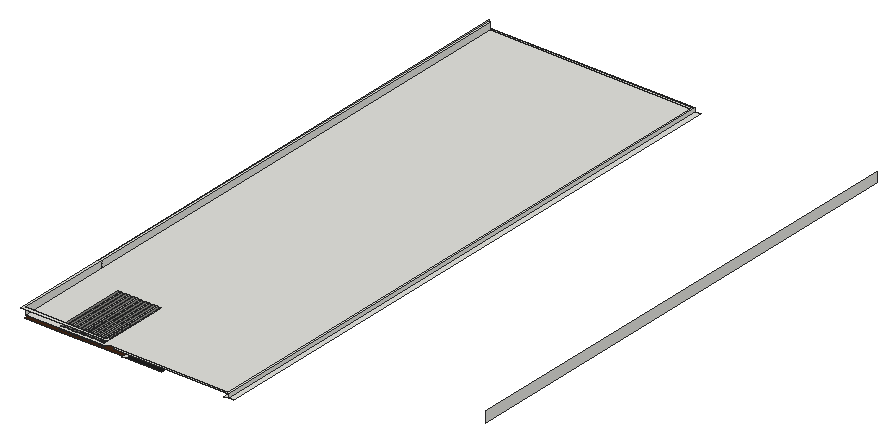
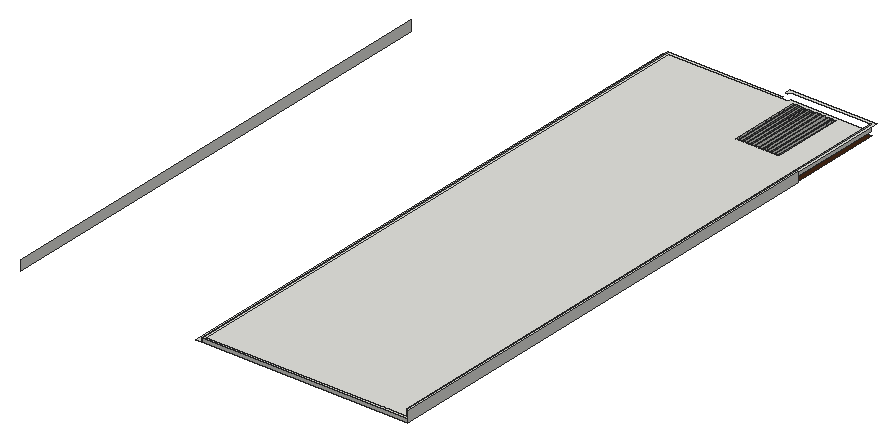
# SketchUp Ruby script. Lengths in inches.
U = 1.inch
M = Sketchup.active_model
def pt(a) = Geom::Point3d.new(a.map { |v| v * U })
def face(e, loops, mat)
  f = e.add_face(loops[0].map { |a| pt(a) })
  loops[1..].each { |l| e.add_face(l.map { |a| pt(a) }).erase! }
  f.material = f.back_material = mat if mat
  f
end
# faces: each face lists its corners as indices into pts; further lists are holes
def faces(e, pts, list, mat = nil) = list.each { |f| face(e, (f[0].is_a?(Array) ? f : [f]).map { |l| l.map { |i| pts[i] } }, mat) }
# xy, xz, yz: faces in a plane at the given z, y or x. An outline is a flat list of corners, or four numbers for a rectangle; further outlines are holes
def ring(l) = l.size == 4 ? [[l[0], l[1]], [l[2], l[1]], [l[2], l[3]], [l[0], l[3]]] : l.each_slice(2).to_a
def flat(e, list, mat, &to3) = list.each { |f| face(e, (f[0].is_a?(Array) ? f : [f]).map { |l| ring(l).map { |u, v| to3.(u, v) } }, mat) }
def xy(e, z, list, mat = nil) = flat(e, list, mat) { |x, y| [x, y, z] }
def xz(e, y, list, mat = nil) = flat(e, list, mat) { |x, z| [x, y, z] }
def yz(e, x, list, mat = nil) = flat(e, list, mat) { |y, z| [x, y, z] }
def lines(e, pts, list) = list.each { |a, b| e.add_line(pt(pts[a]), pt(pts[b])) }
# prism: a flat outline (further loops are holes) pulled along v
def prism(e, loops, v, mat = nil)
  f = face(e, loops, mat); d = Geom::Vector3d.new(v.map { |x| x * U })
  f.pushpull(f.normal.samedirection?(d) ? d.length : -d.length)
end
def box(e, o, s, mat = nil) = prism(e, [[o, [o[0] + s[0], o[1], o[2]], [o[0] + s[0], o[1] + s[1], o[2]], [o[0], o[1] + s[1], o[2]]]], [0, 0, s[2]], mat)
def at(x, y, z, deg = 0) = Geom::Transformation.translation(pt([x, y, z])) * Geom::Transformation.rotation(ORIGIN, Z_AXIS, deg.degrees)
def axes(o, x, y, z) = Geom::Transformation.new([*x, 0, *y, 0, *z, 0, *pt(o).to_a, 1])
def part(name) = M.definitions.add(name)
# library, detail: a bought-in or finely detailed component or shape, given as its bounding box
def library(name, o, s) = part(name).tap { |d| box(d.entities, o, s) }
def detail(e, o, s) = box(e.add_group.entities, o, s)
def put(e, d, t, mat = nil) = e.add_instance(d, t).tap { |i| i.material = mat if mat }
def group(e, t, mat = nil) = e.add_group.tap { |g| g.transformation = t; g.material = mat if mat }.entities
root = M.entities
M.materials.add("[Color M08]").color = [30, 30, 30]
M.materials.add("[Field Square Tile]").color = [211, 167, 108]
M.materials.add("[Granite Light Gray]").color = [149, 148, 144]
M.materials.add("[Wood Veneer 01]").color = [66, 38, 20]
xy(root,380.5,[[676.54,2346.71,676.54,3661.44,228.78,3661.44,228.78,2597.8,444.78,2597.8,444.78,2562.82,218.97,2562.82,218.97,3671.25,686.35,3671.25,686.35,2346.71],[444.78,2346.71,453.7,2425.46],[686.35,2346.71,698.16,3671.25],[444.78,2425.46,444.78,2597.8,228.78,2597.8,228.78,3661.44,676.54,3661.44,676.54,2425.46,629.77,2425.46,629.77,2532.83,534.46,2532.83,534.46,2573.65,453.7,2573.65,453.7,2532.83,445.08,2532.83,445.08,2425.46],[445.08,2425.46,453.7,2532.83],
  [534.46,2425.46,629.77,2532.83],[453.7,2532.83,534.46,2573.65]])
xy(root,380.5,[[453.7,2346.71,534.46,2532.83]],"[Color M08]")
xy(root,380.5,[[[223.8,2347.9,295.73,2562.82],[240.83,2441.63,242.35,2442.01,243.73,2442.76,244.86,2443.84,245.67,2445.18,246.1,2446.6875,246.14,2448.25,245.76,2449.78,245.01,2451.15,243.92,2452.28,242.58,2453.09,241.08,2453.53,239.51,2453.56,237.99,2453.19,236.62,2452.43,235.49,2451.35,234.68,2450.01,234.24,2448.5,234.21,2446.9375,234.58,2445.41,235.34,2444.04,236.42,2442.91,237.76,2442.1,239.27,2441.66],[240.83,2389.88,242.35,2390.26,243.73,2391.01,244.86,2392.09,245.67,2393.43,246.1,2394.9375,246.14,2396.5,245.76,2398.03,245.01,2399.4,243.92,2400.53,242.58,2401.34,241.08,2401.78,239.51,2401.81,237.99,2401.44,236.62,2400.68,235.49,2399.6,234.68,2398.26,234.24,2396.75,234.21,2395.1875,234.58,2393.66,235.34,2392.29,236.42,2391.16,237.76,2390.35,239.27,2389.91],[240.83,2359.13,242.35,2359.51,243.73,2360.26,244.86,2361.34,245.67,2362.68,246.1,2364.1875,246.14,2365.75,245.76,2367.28,245.01,2368.65,243.92,2369.78,242.58,2370.59,241.08,2371.03,239.51,2371.06,237.99,2370.69,236.62,2369.93,235.49,2368.85,234.68,2367.51,234.24,2366,234.21,2364.4375,234.58,2362.91,235.34,2361.54,236.42,2360.41,237.76,2359.6,239.27,2359.16],[240.83,2501.63,242.35,2502.01,243.73,2502.76,244.86,2503.84,245.67,2505.18,246.1,2506.6875,246.14,2508.25,245.76,2509.78,245.01,2511.15,243.92,2512.28,242.58,2513.09,241.08,2513.53,239.51,2513.56,237.99,2513.19,236.62,2512.43,235.49,2511.35,234.68,2510.01,234.24,2508.5,234.21,2506.9375,234.58,2505.41,235.34,2504.04,236.42,2502.91,237.76,2502.1,239.27,2501.66],[280.58,2501.63,282.1,2502.01,283.48,2502.76,284.61,2503.84,285.42,2505.18,285.85,2506.6875,285.89,2508.25,285.51,2509.78,284.76,2511.15,283.67,2512.28,282.33,2513.09,280.83,2513.53,279.26,2513.56,277.74,2513.19,276.37,2512.43,275.24,2511.35,274.43,2510.01,273.99,2508.5,273.96,2506.9375,274.33,2505.41,275.09,2504.04,276.17,2502.91,277.51,2502.1,279.02,2501.66],[280.58,2441.63,282.1,2442.01,283.48,2442.76,284.61,2443.84,285.42,2445.18,285.85,2446.6875,285.89,2448.25,285.51,2449.78,284.76,2451.15,283.67,2452.28,282.33,2453.09,280.83,2453.53,279.26,2453.56,277.74,2453.19,276.37,2452.43,275.24,2451.35,274.43,2450.01,273.99,2448.5,273.96,2446.9375,274.33,2445.41,275.09,2444.04,276.17,2442.91,277.51,2442.1,279.02,2441.66],[280.58,2389.88,282.1,2390.26,283.48,2391.01,284.61,2392.09,285.42,2393.43,285.85,2394.9375,285.89,2396.5,285.51,2398.03,284.76,2399.4,283.67,2400.53,282.33,2401.34,280.83,2401.78,279.26,2401.81,277.74,2401.44,276.37,2400.68,275.24,2399.6,274.43,2398.26,273.99,2396.75,273.96,2395.1875,274.33,2393.66,275.09,2392.29,276.17,2391.16,277.51,2390.35,279.02,2389.91],[280.58,2359.13,282.1,2359.51,283.48,2360.26,284.61,2361.34,285.42,2362.68,285.85,2364.1875,285.89,2365.75,285.51,2367.28,284.76,2368.65,283.67,2369.78,282.33,2370.59,280.83,2371.03,279.26,2371.06,277.74,2370.69,276.37,2369.93,275.24,2368.85,274.43,2367.51,273.99,2366,273.96,2364.4375,274.33,2362.91,275.09,2361.54,276.17,2360.41,277.51,2359.6,279.02,2359.16]],[[295.73,2347.9,444.78,2562.82],[391.18,2355.06,397.43,2516.12],[382.06,2355.06,388.31,2516.12],[372.93,2355.06,379.18,2516.12],[363.81,2355.06,370.06,2516.12],[354.68,2355.06,360.93,2516.12],[345.56,2355.06,351.81,2516.12],[336.43,2355.06,342.68,2516.12],[327.31,2355.06,333.56,2516.12],[318.18,2355.06,324.43,2516.12],[309.06,2355.06,315.31,2516.12],[299.93,2355.06,306.18,2516.12]]],"[Wood Veneer 01]")
xy(root,381.875,[[240.83,2389.88,239.27,2389.91,237.76,2390.35,236.42,2391.16,235.34,2392.29,234.58,2393.66,234.21,2395.1875,234.24,2396.75,234.68,2398.26,235.49,2399.6,236.62,2400.68,237.99,2401.44,239.51,2401.81,241.08,2401.78,242.58,2401.34,243.92,2400.53,245.01,2399.4,245.76,2398.03,246.14,2396.5,246.1,2394.9375,245.67,2393.43,244.86,2392.09,243.73,2391.01,242.35,2390.26],[280.58,2389.88,279.02,2389.91,277.51,2390.35,276.17,2391.16,275.09,2392.29,274.33,2393.66,273.96,2395.1875,273.99,2396.75,274.43,2398.26,275.24,2399.6,276.37,2400.68,277.74,2401.44,279.26,2401.81,280.83,2401.78,282.33,2401.34,283.67,2400.53,284.76,2399.4,285.51,2398.03,285.89,2396.5,285.85,2394.9375,285.42,2393.43,284.61,2392.09,283.48,2391.01,282.1,2390.26],[240.83,2441.63,239.27,2441.66,237.76,2442.1,236.42,2442.91,235.34,2444.04,234.58,2445.41,234.21,2446.9375,234.24,2448.5,234.68,2450.01,235.49,2451.35,236.62,2452.43,237.99,2453.19,239.51,2453.56,241.08,2453.53,242.58,2453.09,243.92,2452.28,245.01,2451.15,245.76,2449.78,246.14,2448.25,246.1,2446.6875,245.67,2445.18,244.86,2443.84,243.73,2442.76,242.35,2442.01],[280.58,2441.63,279.02,2441.66,277.51,2442.1,276.17,2442.91,275.09,2444.04,274.33,2445.41,273.96,2446.9375,273.99,2448.5,274.43,2450.01,275.24,2451.35,276.37,2452.43,277.74,2453.19,279.26,2453.56,280.83,2453.53,282.33,2453.09,283.67,2452.28,284.76,2451.15,285.51,2449.78,285.89,2448.25,285.85,2446.6875,285.42,2445.18,284.61,2443.84,283.48,2442.76,282.1,2442.01],[240.83,2501.63,239.27,2501.66,237.76,2502.1,236.42,2502.91,235.34,2504.04,234.58,2505.41,234.21,2506.9375,234.24,2508.5,234.68,2510.01,235.49,2511.35,236.62,2512.43,237.99,2513.19,239.51,2513.56,241.08,2513.53,242.58,2513.09,243.92,2512.28,245.01,2511.15,245.76,2509.78,246.14,2508.25,246.1,2506.6875,245.67,2505.18,244.86,2503.84,243.73,2502.76,242.35,2502.01],
  [280.58,2501.63,279.02,2501.66,277.51,2502.1,276.17,2502.91,275.09,2504.04,274.33,2505.41,273.96,2506.9375,273.99,2508.5,274.43,2510.01,275.24,2511.35,276.37,2512.43,277.74,2513.19,279.26,2513.56,280.83,2513.53,282.33,2513.09,283.67,2512.28,284.76,2511.15,285.51,2509.78,285.89,2508.25,285.85,2506.6875,285.42,2505.18,284.61,2503.84,283.48,2502.76,282.1,2502.01]],"[Field Square Tile]")
xy(root,388.625,[[[225.31,2346.49,408.63,2346.49,408.63,2353.05,680,2353.05,680,3664.91,225.31,3664.91],[299.93,2355.06,306.18,2516.12],[309.06,2355.06,315.31,2516.12],[318.18,2355.06,324.43,2516.12],[327.31,2355.06,333.56,2516.12],[336.43,2355.06,342.68,2516.12],[345.56,2355.06,351.81,2516.12],[354.68,2355.06,360.93,2516.12],[363.81,2355.06,370.06,2516.12],[372.93,2355.06,379.18,2516.12],[382.06,2355.06,388.31,2516.12],[391.18,2355.06,397.43,2516.12]],[425.6875,2346.71,686.35,2346.71,686.35,3671.25,218.97,3671.25,225.31,3664.91,680,3664.91,680,2353.05,425.6875,2353.05]])
xy(root,403.8125,[[218.97,2340.15,414.98,2340.15,414.98,2353.05,408.63,2353.05,408.63,2346.49,225.31,2346.49,225.31,3664.91,218.97,3671.25]])
xz(root,2516.12,[[299.93,380.5,306.18,388.625],[309.06,380.5,315.31,388.625],[318.18,380.5,324.43,388.625],[327.31,380.5,333.56,388.625],[336.43,380.5,342.68,388.625],
  [345.56,380.5,351.81,388.625],[354.68,380.5,360.93,388.625],[363.81,380.5,370.06,388.625],[372.93,380.5,379.18,388.625],[382.06,380.5,388.31,388.625],
  [391.18,380.5,397.43,388.625]],"[Granite Light Gray]")
xz(root,3671.25,[[218.97,380.5,686.35,388.625]])
yz(root,218.97,[[2562.82,380.5,3671.25,403.8125]])
yz(root,225.31,[[2346.49,388.625,2562.82,403.8125],[2562.82,388.625,3664.91,403.8125]])
yz(root,299.93,[[2355.06,380.5,2516.12,388.625]],"[Granite Light Gray]")
yz(root,306.18,[[2355.06,380.5,2516.12,388.625]])
yz(root,309.06,[[2355.06,380.5,2516.12,388.625]],"[Granite Light Gray]")
yz(root,315.31,[[2355.06,380.5,2516.12,388.625]])
yz(root,318.18,[[2355.06,380.5,2516.12,388.625]],"[Granite Light Gray]")
yz(root,324.43,[[2355.06,380.5,2516.12,388.625]])
yz(root,327.31,[[2355.06,380.5,2516.12,388.625]],"[Granite Light Gray]")
yz(root,333.56,[[2355.06,380.5,2516.12,388.625]])
yz(root,336.43,[[2355.06,380.5,2516.12,388.625]],"[Granite Light Gray]")
yz(root,342.68,[[2355.06,380.5,2516.12,388.625]])
yz(root,345.56,[[2355.06,380.5,2516.12,388.625]],"[Granite Light Gray]")
yz(root,351.81,[[2355.06,380.5,2516.12,388.625]])
yz(root,354.68,[[2355.06,380.5,2516.12,388.625]],"[Granite Light Gray]")
yz(root,360.93,[[2355.06,380.5,2516.12,388.625]])
yz(root,363.81,[[2355.06,380.5,2516.12,388.625]],"[Granite Light Gray]")
yz(root,370.06,[[2355.06,380.5,2516.12,388.625]])
yz(root,372.93,[[2355.06,380.5,2516.12,388.625]],"[Granite Light Gray]")
yz(root,379.18,[[2355.06,380.5,2516.12,388.625]])
yz(root,382.06,[[2355.06,380.5,2516.12,388.625]],"[Granite Light Gray]")
yz(root,388.31,[[2355.06,380.5,2516.12,388.625]])
yz(root,391.18,[[2355.06,380.5,2516.12,388.625]],"[Granite Light Gray]")
yz(root,397.43,[[2355.06,380.5,2516.12,388.625]])
yz(root,686.35,[[2346.71,380.5,3671.25,388.625]])
yz(root,1097.72,[[2562.82,380.5,3671.25,403.8125]])
p = [[239.27,2389.91,380.5],[237.76,2390.35,380.5],[237.76,2390.35,381.875],[239.27,2389.91,381.875],[240.83,2389.88,380.5],[240.83,2389.88,381.875],
  [242.35,2390.26,380.5],[242.35,2390.26,381.875],[279.02,2389.91,380.5],[277.51,2390.35,380.5],[277.51,2390.35,381.875],[279.02,2389.91,381.875],
  [280.58,2389.88,380.5],[280.58,2389.88,381.875],[282.1,2390.26,380.5],[282.1,2390.26,381.875],[243.73,2391.01,380.5],[243.73,2391.01,381.875],
  [283.48,2391.01,380.5],[283.48,2391.01,381.875],[236.42,2391.16,380.5],[236.42,2391.16,381.875],[276.17,2391.16,380.5],[276.17,2391.16,381.875],
  [244.86,2392.09,380.5],[244.86,2392.09,381.875],[284.61,2392.09,380.5],[284.61,2392.09,381.875],[235.34,2392.29,380.5],[235.34,2392.29,381.875],
  [275.09,2392.29,380.5],[275.09,2392.29,381.875],[245.67,2393.43,380.5],[245.67,2393.43,381.875],[285.42,2393.43,380.5],[285.42,2393.43,381.875],
  [234.58,2393.66,380.5],[234.58,2393.66,381.875],[274.33,2393.66,380.5],[274.33,2393.66,381.875],[246.1,2394.9375,380.5],[246.1,2394.9375,381.875],
  [285.85,2394.9375,380.5],[285.85,2394.9375,381.875],[234.21,2395.1875,380.5],[234.21,2395.1875,381.875],[273.96,2395.1875,380.5],[273.96,2395.1875,381.875],
  [246.14,2396.5,380.5],[246.14,2396.5,381.875],[285.89,2396.5,380.5],[285.89,2396.5,381.875],[234.24,2396.75,380.5],[234.24,2396.75,381.875],
  [273.99,2396.75,380.5],[273.99,2396.75,381.875],[245.76,2398.03,380.5],[245.76,2398.03,381.875],[285.51,2398.03,380.5],[285.51,2398.03,381.875],
  [234.68,2398.26,380.5],[234.68,2398.26,381.875],[274.43,2398.26,380.5],[274.43,2398.26,381.875],[245.01,2399.4,380.5],[245.01,2399.4,381.875],
  [284.76,2399.4,380.5],[284.76,2399.4,381.875],[235.49,2399.6,380.5],[235.49,2399.6,381.875],[275.24,2399.6,380.5],[275.24,2399.6,381.875],
  [243.92,2400.53,380.5],[243.92,2400.53,381.875],[283.67,2400.53,380.5],[283.67,2400.53,381.875],[236.62,2400.68,380.5],[236.62,2400.68,381.875],
  [276.37,2400.68,380.5],[276.37,2400.68,381.875],[242.58,2401.34,380.5],[242.58,2401.34,381.875],[282.33,2401.34,380.5],[282.33,2401.34,381.875],
  [237.99,2401.44,380.5],[237.99,2401.44,381.875],[277.74,2401.44,380.5],[277.74,2401.44,381.875],[241.08,2401.78,380.5],[241.08,2401.78,381.875],
  [280.83,2401.78,380.5],[280.83,2401.78,381.875],[239.51,2401.81,380.5],[239.51,2401.81,381.875],[279.26,2401.81,380.5],[279.26,2401.81,381.875],
  [240.83,2441.63,380.5],[239.27,2441.66,380.5],[239.27,2441.66,381.875],[240.83,2441.63,381.875],[242.35,2442.01,380.5],[242.35,2442.01,381.875],
  [280.58,2441.63,380.5],[279.02,2441.66,380.5],[279.02,2441.66,381.875],[280.58,2441.63,381.875],[282.1,2442.01,380.5],[282.1,2442.01,381.875],
  [237.76,2442.1,380.5],[237.76,2442.1,381.875],[277.51,2442.1,380.5],[277.51,2442.1,381.875],[243.73,2442.76,380.5],[243.73,2442.76,381.875],
  [283.48,2442.76,380.5],[283.48,2442.76,381.875],[236.42,2442.91,380.5],[236.42,2442.91,381.875],[276.17,2442.91,380.5],[276.17,2442.91,381.875],
  [244.86,2443.84,380.5],[244.86,2443.84,381.875],[284.61,2443.84,380.5],[284.61,2443.84,381.875],[235.34,2444.04,380.5],[235.34,2444.04,381.875],
  [275.09,2444.04,380.5],[275.09,2444.04,381.875],[245.67,2445.18,380.5],[245.67,2445.18,381.875],[285.42,2445.18,380.5],[285.42,2445.18,381.875],
  [234.58,2445.41,380.5],[234.58,2445.41,381.875],[274.33,2445.41,380.5],[274.33,2445.41,381.875],[246.1,2446.6875,380.5],[246.1,2446.6875,381.875],
  [285.85,2446.6875,380.5],[285.85,2446.6875,381.875],[234.21,2446.9375,380.5],[234.21,2446.9375,381.875],[273.96,2446.9375,380.5],[273.96,2446.9375,381.875],
  [246.14,2448.25,380.5],[246.14,2448.25,381.875],[285.89,2448.25,380.5],[285.89,2448.25,381.875],[234.24,2448.5,380.5],[234.24,2448.5,381.875],
  [273.99,2448.5,380.5],[273.99,2448.5,381.875],[245.76,2449.78,380.5],[245.76,2449.78,381.875],[285.51,2449.78,380.5],[285.51,2449.78,381.875],
  [234.68,2450.01,380.5],[234.68,2450.01,381.875],[274.43,2450.01,380.5],[274.43,2450.01,381.875],[245.01,2451.15,380.5],[245.01,2451.15,381.875],
  [284.76,2451.15,380.5],[284.76,2451.15,381.875],[235.49,2451.35,380.5],[235.49,2451.35,381.875],[275.24,2451.35,380.5],[275.24,2451.35,381.875],
  [243.92,2452.28,380.5],[243.92,2452.28,381.875],[283.67,2452.28,380.5],[283.67,2452.28,381.875],[236.62,2452.43,380.5],[236.62,2452.43,381.875],
  [276.37,2452.43,380.5],[276.37,2452.43,381.875],[242.58,2453.09,380.5],[242.58,2453.09,381.875],[282.33,2453.09,380.5],[282.33,2453.09,381.875],
  [237.99,2453.19,380.5],[237.99,2453.19,381.875],[277.74,2453.19,380.5],[277.74,2453.19,381.875],[241.08,2453.53,380.5],[241.08,2453.53,381.875],
  [280.83,2453.53,380.5],[280.83,2453.53,381.875],[239.51,2453.56,380.5],[239.51,2453.56,381.875],[279.26,2453.56,380.5],[279.26,2453.56,381.875],
  [240.83,2501.63,380.5],[239.27,2501.66,380.5],[239.27,2501.66,381.875],[240.83,2501.63,381.875],[242.35,2502.01,380.5],[242.35,2502.01,381.875],
  [280.58,2501.63,380.5],[279.02,2501.66,380.5],[279.02,2501.66,381.875],[280.58,2501.63,381.875],[282.1,2502.01,380.5],[282.1,2502.01,381.875],
  [237.76,2502.1,380.5],[237.76,2502.1,381.875],[277.51,2502.1,380.5],[277.51,2502.1,381.875],[243.73,2502.76,380.5],[243.73,2502.76,381.875],
  [283.48,2502.76,380.5],[283.48,2502.76,381.875],[236.42,2502.91,380.5],[236.42,2502.91,381.875],[276.17,2502.91,380.5],[276.17,2502.91,381.875],
  [244.86,2503.84,380.5],[244.86,2503.84,381.875],[284.61,2503.84,380.5],[284.61,2503.84,381.875],[235.34,2504.04,380.5],[235.34,2504.04,381.875],
  [275.09,2504.04,380.5],[275.09,2504.04,381.875],[245.67,2505.18,380.5],[245.67,2505.18,381.875],[285.42,2505.18,380.5],[285.42,2505.18,381.875],
  [234.58,2505.41,380.5],[234.58,2505.41,381.875],[274.33,2505.41,380.5],[274.33,2505.41,381.875],[246.1,2506.6875,380.5],[246.1,2506.6875,381.875],
  [285.85,2506.6875,380.5],[285.85,2506.6875,381.875],[234.21,2506.9375,380.5],[234.21,2506.9375,381.875],[273.96,2506.9375,380.5],[273.96,2506.9375,381.875],
  [246.14,2508.25,380.5],[246.14,2508.25,381.875],[285.89,2508.25,380.5],[285.89,2508.25,381.875],[234.24,2508.5,380.5],[234.24,2508.5,381.875],
  [273.99,2508.5,380.5],[273.99,2508.5,381.875],[245.76,2509.78,380.5],[245.76,2509.78,381.875],[285.51,2509.78,380.5],[285.51,2509.78,381.875],
  [234.68,2510.01,380.5],[234.68,2510.01,381.875],[274.43,2510.01,380.5],[274.43,2510.01,381.875],[245.01,2511.15,380.5],[245.01,2511.15,381.875],
  [284.76,2511.15,380.5],[284.76,2511.15,381.875],[235.49,2511.35,380.5],[235.49,2511.35,381.875],[275.24,2511.35,380.5],[275.24,2511.35,381.875],
  [243.92,2512.28,380.5],[243.92,2512.28,381.875],[283.67,2512.28,380.5],[283.67,2512.28,381.875],[236.62,2512.43,380.5],[236.62,2512.43,381.875],
  [276.37,2512.43,380.5],[276.37,2512.43,381.875],[242.58,2513.09,380.5],[242.58,2513.09,381.875],[282.33,2513.09,380.5],[282.33,2513.09,381.875],
  [237.99,2513.19,380.5],[237.99,2513.19,381.875],[277.74,2513.19,380.5],[277.74,2513.19,381.875],[241.08,2513.53,380.5],[241.08,2513.53,381.875],
  [280.83,2513.53,380.5],[280.83,2513.53,381.875],[239.51,2513.56,380.5],[239.51,2513.56,381.875],[279.26,2513.56,380.5],[279.26,2513.56,381.875],
  [225.31,3664.91,388.625],[218.97,3671.25,388.625],[218.97,3671.25,403.8125],[225.31,3664.91,403.8125]]
faces(root,p,[[0,1,2,3],[4,0,3,5],[6,4,5,7],[8,9,10,11],[12,8,11,13],[14,12,13,15],[16,6,7,17],[18,14,15,19],
  [1,20,21,2],[9,22,23,10],[24,16,17,25],[26,18,19,27],[20,28,29,21],[22,30,31,23],[32,24,25,33],[34,26,27,35],
  [28,36,37,29],[30,38,39,31],[40,32,33,41],[42,34,35,43],[36,44,45,37],[38,46,47,39],[48,40,41,49],[50,42,43,51],
  [44,52,53,45],[46,54,55,47],[56,48,49,57],[58,50,51,59],[52,60,61,53],[54,62,63,55],[64,56,57,65],[66,58,59,67],
  [60,68,69,61],[62,70,71,63],[72,64,65,73],[74,66,67,75],[68,76,77,69],[70,78,79,71],[80,72,73,81],[82,74,75,83],
  [76,84,85,77],[78,86,87,79],[88,80,81,89],[90,82,83,91],[84,92,93,85],[86,94,95,87],[92,88,89,93],[94,90,91,95],
  [96,97,98,99],[100,96,99,101],[102,103,104,105],[106,102,105,107],[97,108,109,98],[103,110,111,104],[112,100,101,113],[114,106,107,115],
  [108,116,117,109],[110,118,119,111],[120,112,113,121],[122,114,115,123],[116,124,125,117],[118,126,127,119],[128,120,121,129],[130,122,123,131],
  [124,132,133,125],[126,134,135,127],[136,128,129,137],[138,130,131,139],[132,140,141,133],[134,142,143,135],[144,136,137,145],[146,138,139,147],
  [140,148,149,141],[142,150,151,143],[152,144,145,153],[154,146,147,155],[148,156,157,149],[150,158,159,151],[160,152,153,161],[162,154,155,163],
  [156,164,165,157],[158,166,167,159],[168,160,161,169],[170,162,163,171],[164,172,173,165],[166,174,175,167],[176,168,169,177],[178,170,171,179],
  [172,180,181,173],[174,182,183,175],[184,176,177,185],[186,178,179,187],[180,188,189,181],[182,190,191,183],[188,184,185,189],[190,186,187,191],
  [192,193,194,195],[196,192,195,197],[198,199,200,201],[202,198,201,203],[193,204,205,194],[199,206,207,200],[208,196,197,209],[210,202,203,211],
  [204,212,213,205],[206,214,215,207],[216,208,209,217],[218,210,211,219],[212,220,221,213],[214,222,223,215],[224,216,217,225],[226,218,219,227],
  [220,228,229,221],[222,230,231,223],[232,224,225,233],[234,226,227,235],[228,236,237,229],[230,238,239,231],[240,232,233,241],[242,234,235,243],
  [236,244,245,237],[238,246,247,239],[248,240,241,249],[250,242,243,251],[244,252,253,245],[246,254,255,247],[256,248,249,257],[258,250,251,259],
  [252,260,261,253],[254,262,263,255],[264,256,257,265],[266,258,259,267],[260,268,269,261],[262,270,271,263],[272,264,265,273],[274,266,267,275],
  [268,276,277,269],[270,278,279,271],[280,272,273,281],[282,274,275,283],[276,284,285,277],[278,286,287,279],[284,280,281,285],[286,282,283,287]],"[Field Square Tile]")
faces(root,p,[[288,289,290,291]])
